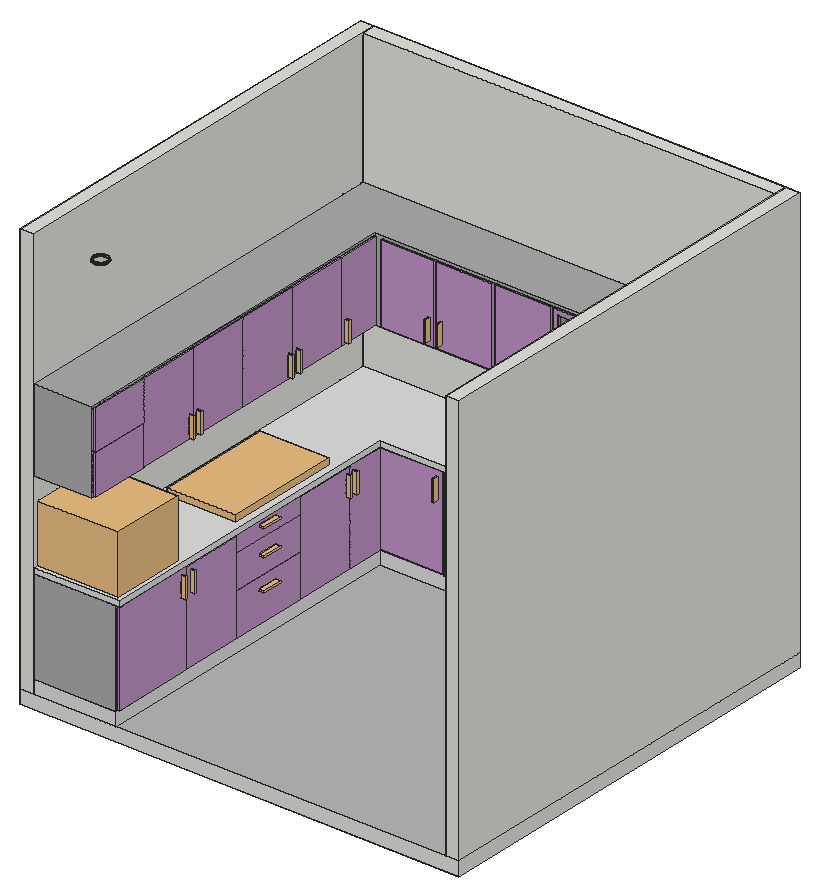
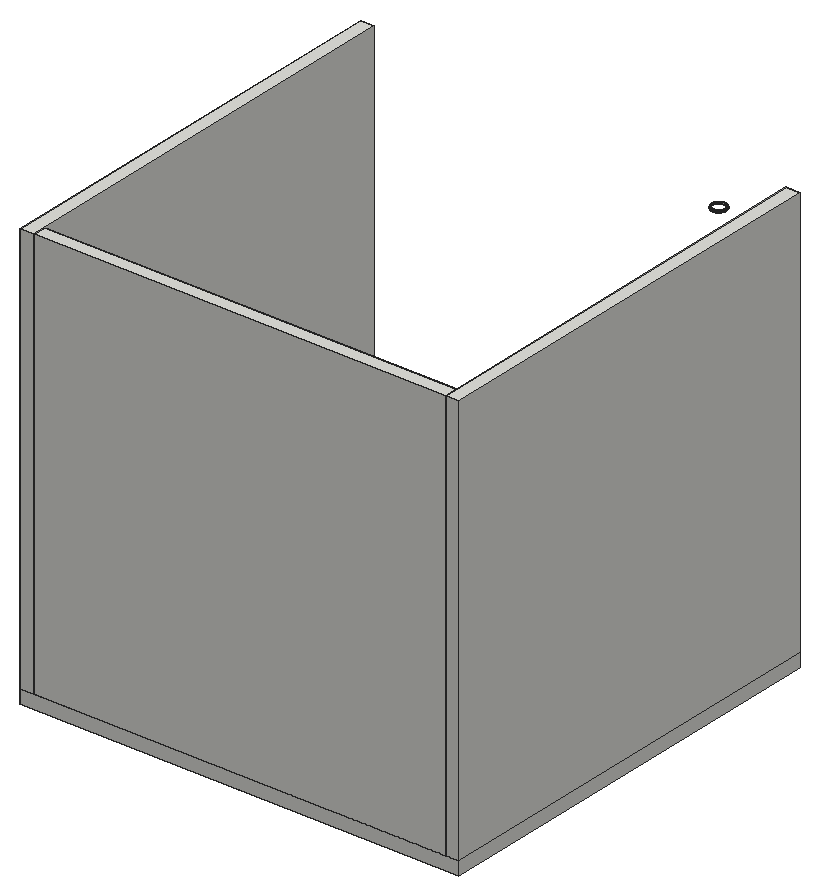
# SketchUp Ruby script. Lengths in inches.
U = 1.inch
M = Sketchup.active_model
def pt(a) = Geom::Point3d.new(a.map { |v| v * U })
def face(e, loops, mat)
  f = e.add_face(loops[0].map { |a| pt(a) })
  loops[1..].each { |l| e.add_face(l.map { |a| pt(a) }).erase! }
  f.material = f.back_material = mat if mat
  f
end
# faces: each face lists its corners as indices into pts; further lists are holes
def faces(e, pts, list, mat = nil) = list.each { |f| face(e, (f[0].is_a?(Array) ? f : [f]).map { |l| l.map { |i| pts[i] } }, mat) }
# xy, xz, yz: faces in a plane at the given z, y or x. An outline is a flat list of corners, or four numbers for a rectangle; further outlines are holes
def ring(l) = l.size == 4 ? [[l[0], l[1]], [l[2], l[1]], [l[2], l[3]], [l[0], l[3]]] : l.each_slice(2).to_a
def flat(e, list, mat, &to3) = list.each { |f| face(e, (f[0].is_a?(Array) ? f : [f]).map { |l| ring(l).map { |u, v| to3.(u, v) } }, mat) }
def xy(e, z, list, mat = nil) = flat(e, list, mat) { |x, y| [x, y, z] }
def xz(e, y, list, mat = nil) = flat(e, list, mat) { |x, z| [x, y, z] }
def yz(e, x, list, mat = nil) = flat(e, list, mat) { |y, z| [x, y, z] }
def lines(e, pts, list) = list.each { |a, b| e.add_line(pt(pts[a]), pt(pts[b])) }
# prism: a flat outline (further loops are holes) pulled along v
def prism(e, loops, v, mat = nil)
  f = face(e, loops, mat); d = Geom::Vector3d.new(v.map { |x| x * U })
  f.pushpull(f.normal.samedirection?(d) ? d.length : -d.length)
end
def box(e, o, s, mat = nil) = prism(e, [[o, [o[0] + s[0], o[1], o[2]], [o[0] + s[0], o[1] + s[1], o[2]], [o[0], o[1] + s[1], o[2]]]], [0, 0, s[2]], mat)
def at(x, y, z, deg = 0) = Geom::Transformation.translation(pt([x, y, z])) * Geom::Transformation.rotation(ORIGIN, Z_AXIS, deg.degrees)
def axes(o, x, y, z) = Geom::Transformation.new([*x, 0, *y, 0, *z, 0, *pt(o).to_a, 1])
def part(name) = M.definitions.add(name)
# library, detail: a bought-in or finely detailed component or shape, given as its bounding box
def library(name, o, s) = part(name).tap { |d| box(d.entities, o, s) }
def detail(e, o, s) = box(e.add_group.entities, o, s)
def put(e, d, t, mat = nil) = e.add_instance(d, t).tap { |i| i.material = mat if mat }
def group(e, t, mat = nil) = e.add_group.tap { |g| g.transformation = t; g.material = mat if mat }.entities
root = M.entities
M.materials.add("Marble White 100cm").color = [222, 222, 222]
M.materials.add("Tiles Simple 02 100cm").color = [183, 183, 183]
M.materials.add("base cabinate colour").color = [192, 148, 199]
M.materials.add("cabinate colour").color = [171, 171, 171]
M.materials.add("clear glass").color = [0, 0, 0]
M.materials["clear glass"].alpha = 0.1
c1 = library("geladeira side by side",[0,0,0],[32.68,30.71,73.23])
c2 = library("9-POIGNEE CLC2",[-3.01,-0.26,0],[6.02,0.52,1.49])
c3 = library("Kitchen sink assembly",[0,0,0],[21.65,23.57,24.55])
c4 = library("Group\#38",[0,0,0],[9.87,6.84,12.32])
c5 = library("7-TABLE DE CUISSON CLC2",[-16.93,-10.04,0.13],[33.86,20.08,1.97])
xy(root,113.9,[[[16.806,6.374,16.577,6.375,16.349,6.4,16.125,6.449,15.907,6.521,15.697,6.616,15.499,6.732,15.315,6.868,15.145,7.023,14.992,7.194,14.858,7.381,14.745,7.58,14.653,7.79,14.583,8.009,14.537,8.234,14.514,8.462,14.515,8.692,14.541,8.92,14.59,9.144,14.662,9.362,14.757,9.571,14.872,9.769,15.008,9.954,15.163,10.124,15.335,10.276,15.521,10.41,15.72,10.524,15.931,10.616,16.149,10.685,16.374,10.732,16.603,10.754,16.832,10.753,17.06,10.728,17.284,10.679,17.502,10.607,17.711,10.512,17.91,10.396,18.094,10.26,18.264,10.105,18.417,9.934,18.551,9.747,18.664,9.548,18.756,9.338,18.826,9.119,18.872,8.894,18.895,8.666,18.894,8.436,18.868,8.208,18.819,7.984,18.747,7.766,18.652,7.557,18.537,7.359,18.4,7.174,18.246,7.004,18.074,6.852,17.888,6.718,17.689,6.604,17.478,6.512,17.26,6.443,17.035,6.396],[16.797,6.573,16.901,6.584,17.005,6.594,17.209,6.636,17.308,6.668,17.408,6.699,17.503,6.741,17.599,6.783,17.689,6.835,17.78,6.886,17.865,6.947,17.949,7.008,18.027,7.077,18.105,7.147,18.176,7.224,18.246,7.301,18.308,7.385,18.369,7.469,18.475,7.649,18.561,7.839,18.594,7.938,18.626,8.037,18.649,8.139,18.671,8.241,18.682,8.344,18.694,8.448,18.695,8.552,18.695,8.657,18.685,8.76,18.675,8.864,18.653,8.966,18.632,9.068,18.601,9.168,18.569,9.267,18.527,9.363,18.485,9.458,18.434,9.549,18.382,9.64,18.321,9.724,18.261,9.809,18.191,9.887,18.122,9.965,17.968,10.105,17.8,10.229,17.71,10.282,17.62,10.334,17.43,10.42,17.232,10.486,17.028,10.53,16.924,10.542,16.82,10.553,16.612,10.555,16.508,10.544,16.404,10.534,16.2,10.492,16.101,10.46,16.001,10.429,15.906,10.387,15.81,10.345,15.72,10.293,15.629,10.242,15.459,10.12,15.382,10.051,15.304,9.981,15.233,9.904,15.163,9.827,15.101,9.743,15.04,9.659,14.934,9.479,14.848,9.289,14.815,9.19,14.783,9.091,14.76,8.989,14.738,8.887,14.727,8.784,14.715,8.68,14.714,8.576,14.714,8.471,14.724,8.368,14.734,8.264,14.755,8.162,14.777,8.06,14.808,7.96,14.84,7.861,14.882,7.765,14.924,7.67,14.975,7.579,15.027,7.488,15.088,7.404,15.148,7.319,15.218,7.241,15.287,7.163,15.441,7.023,15.609,6.899,15.699,6.846,15.789,6.794,15.979,6.708,16.177,6.642,16.381,6.598,16.485,6.586,16.588,6.575,16.693,6.574]],[16.797,6.573,16.693,6.574,16.901,6.584],[16.693,6.574,16.588,6.575,16.485,6.586],[16.901,6.584,17.107,6.615,17.005,6.594],[16.485,6.586,16.381,6.598,16.279,6.62],
  [17.107,6.615,17.308,6.668,17.209,6.636],[16.279,6.62,16.177,6.642,16.078,6.675],[17.308,6.668,17.503,6.741,17.408,6.699],[16.078,6.675,15.979,6.708,15.884,6.751],[17.503,6.741,17.689,6.835,17.599,6.783],
  [15.884,6.751,15.789,6.794,15.699,6.846],[17.689,6.835,17.865,6.947,17.78,6.886],[15.699,6.846,15.609,6.899,15.525,6.961],[17.865,6.947,18.027,7.077,17.949,7.008],[15.525,6.961,15.441,7.023,15.364,7.093],
  [18.027,7.077,18.176,7.224,18.105,7.147],[15.364,7.093,15.287,7.163,15.218,7.241],[18.176,7.224,18.308,7.385,18.246,7.301],[15.218,7.241,15.148,7.319,15.088,7.404],[18.308,7.385,18.422,7.559,18.369,7.469],
  [15.088,7.404,15.027,7.488,14.975,7.579],[18.422,7.559,18.518,7.744,18.475,7.649],[14.975,7.579,14.924,7.67,14.882,7.765],[18.518,7.744,18.594,7.938,18.561,7.839],[14.882,7.765,14.84,7.861,14.808,7.96],
  [18.594,7.938,18.649,8.139,18.626,8.037],[14.808,7.96,14.777,8.06,14.755,8.162],[14.755,8.162,14.734,8.264,14.724,8.368],[14.724,8.368,14.714,8.471,14.714,8.576],[14.714,8.576,14.715,8.68,14.727,8.784],
  [14.727,8.784,14.738,8.887,14.76,8.989],[14.76,8.989,14.783,9.091,14.815,9.19],[14.815,9.19,14.848,9.289,14.891,9.384],[14.891,9.384,14.934,9.479,14.987,9.569],[14.987,9.569,15.04,9.659,15.101,9.743],
  [15.101,9.743,15.163,9.827,15.233,9.904],[15.233,9.904,15.304,9.981,15.382,10.051],[15.382,10.051,15.459,10.12,15.544,10.181],[15.544,10.181,15.629,10.242,15.72,10.293],[15.72,10.293,15.81,10.345,15.906,10.387]])
p = [[16.125,6.449,114],[15.907,6.521,114],[15.907,6.521,113.9],[16.125,6.449,113.9],[16.349,6.4,114],[16.349,6.4,113.9],
  [16.577,6.375,114],[16.577,6.375,113.9],[16.806,6.374,114],[16.806,6.374,113.9],[17.035,6.396,114],[17.035,6.396,113.9],
  [17.26,6.443,114],[17.26,6.443,113.9],[17.478,6.512,114],[17.478,6.512,113.9],[15.697,6.616,114],[15.697,6.616,113.9],
  [17.689,6.604,114],[17.689,6.604,113.9],[15.499,6.732,114],[15.499,6.732,113.9],[16.177,6.642,114.472],[16.177,6.642,113.9],
  [16.078,6.675,113.9],[15.979,6.708,113.9],[15.979,6.708,114.472],[16.381,6.598,114.472],[16.381,6.598,113.9],[16.279,6.62,113.9],
  [16.588,6.575,114.472],[16.588,6.575,113.9],[16.485,6.586,113.9],[16.797,6.573,114.472],[16.797,6.573,113.9],[16.693,6.574,113.9],
  [17.005,6.594,114.472],[17.005,6.594,113.9],[16.901,6.584,113.9],[17.209,6.636,114.472],[17.209,6.636,113.9],[17.107,6.615,113.9],
  [17.408,6.699,114.472],[17.408,6.699,113.9],[17.308,6.668,113.9],[17.888,6.718,114],[17.888,6.718,113.9],[15.315,6.868,114],
  [15.315,6.868,113.9],[15.884,6.751,113.9],[15.789,6.794,113.9],[15.789,6.794,114.472],[17.599,6.783,114.472],[17.599,6.783,113.9],
  [17.503,6.741,113.9],[18.074,6.852,114],[18.074,6.852,113.9],[15.699,6.846,113.9],[15.609,6.899,113.9],[15.609,6.899,114.472],
  [17.78,6.886,114.472],[17.78,6.886,113.9],[17.689,6.835,113.9],[15.145,7.023,114],[15.145,7.023,113.9],[15.525,6.961,113.9],
  [15.441,7.023,113.9],[15.441,7.023,114.472],[17.949,7.008,114.472],[17.949,7.008,113.9],[17.865,6.947,113.9],[18.246,7.004,114],
  [18.246,7.004,113.9],[14.992,7.194,114],[14.992,7.194,113.9],[15.364,7.093,113.9],[15.287,7.163,113.9],[15.287,7.163,114.472],
  [18.105,7.147,114.472],[18.105,7.147,113.9],[18.027,7.077,113.9],[18.4,7.174,114],[18.4,7.174,113.9],[18.246,7.301,114.472],
  [18.246,7.301,113.9],[18.176,7.224,113.9],[14.858,7.381,114],[14.858,7.381,113.9],[15.218,7.241,113.9],[15.148,7.319,113.9],
  [15.148,7.319,114.472],[18.537,7.359,114],[18.537,7.359,113.9],[15.088,7.404,113.9],[15.027,7.488,113.9],[15.027,7.488,114.472],
  [18.369,7.469,114.472],[18.369,7.469,113.9],[18.308,7.385,113.9],[14.745,7.58,114],[14.745,7.58,113.9],[18.652,7.557,114],
  [18.652,7.557,113.9],[14.975,7.579,113.9],[14.924,7.67,113.9],[14.924,7.67,114.472],[18.475,7.649,114.472],[18.475,7.649,113.9],
  [18.422,7.559,113.9],[14.653,7.79,114],[14.653,7.79,113.9],[18.561,7.839,114.472],[18.561,7.839,113.9],[18.518,7.744,113.9],
  [18.747,7.766,114],[18.747,7.766,113.9],[14.882,7.765,113.9],[14.84,7.861,113.9],[14.84,7.861,114.472],[14.583,8.009,114],
  [14.583,8.009,113.9],[18.626,8.037,114.472],[18.626,8.037,113.9],[18.594,7.938,113.9],[18.819,7.984,114],[18.819,7.984,113.9],
  [14.808,7.96,113.9],[14.777,8.06,113.9],[14.777,8.06,114.472],[14.537,8.234,114],[14.537,8.234,113.9],[18.671,8.241,114.472],
  [18.671,8.241,113.9],[18.649,8.139,113.9],[18.868,8.208,114],[18.868,8.208,113.9],[14.755,8.162,113.9],[14.734,8.264,113.9],
  [14.734,8.264,114.472],[14.514,8.462,114],[14.514,8.462,113.9],[18.694,8.448,114.472],[18.694,8.448,113.9],[18.682,8.344,113.9],
  [18.894,8.436,114],[18.894,8.436,113.9],[14.724,8.368,113.9],[14.714,8.471,113.9],[14.714,8.471,114.472],[18.695,8.657,114.472],
  [18.695,8.657,113.9],[18.695,8.552,113.9],[18.895,8.666,114],[18.895,8.666,113.9],[14.515,8.692,114],[14.515,8.692,113.9],
  [14.714,8.576,113.9],[14.715,8.68,113.9],[14.715,8.68,114.472],[14.541,8.92,114],[14.541,8.92,113.9],[14.727,8.784,113.9],
  [14.738,8.887,113.9],[14.738,8.887,114.472],[18.675,8.864,114.472],[18.675,8.864,113.9],[18.685,8.76,113.9],[18.872,8.894,114],
  [18.872,8.894,113.9],[14.59,9.144,114],[14.59,9.144,113.9],[14.76,8.989,113.9],[14.783,9.091,113.9],[14.783,9.091,114.472],
  [18.632,9.068,114.472],[18.632,9.068,113.9],[18.653,8.966,113.9],[18.826,9.119,114],[18.826,9.119,113.9],[14.662,9.362,114],
  [14.662,9.362,113.9],[14.815,9.19,113.9],[14.848,9.289,113.9],[14.848,9.289,114.472],[18.569,9.267,114.472],[18.569,9.267,113.9],
  [18.601,9.168,113.9],[18.756,9.338,114],[18.756,9.338,113.9],[14.891,9.384,113.9],[14.934,9.479,113.9],[14.934,9.479,114.472],
  [18.485,9.458,114.472],[18.485,9.458,113.9],[18.527,9.363,113.9],[18.664,9.548,114],[18.664,9.548,113.9],[14.757,9.571,114],
  [14.757,9.571,113.9],[14.987,9.569,113.9],[15.04,9.659,113.9],[15.04,9.659,114.472],[18.382,9.64,114.472],[18.382,9.64,113.9],
  [18.434,9.549,113.9],[18.551,9.747,114],[18.551,9.747,113.9],[14.872,9.769,114],[14.872,9.769,113.9],[18.261,9.809,114.472],
  [18.261,9.809,113.9],[18.321,9.724,113.9],[15.101,9.743,113.9],[15.163,9.827,113.9],[15.163,9.827,114.472],[18.417,9.934,114],
  [18.417,9.934,113.9],[15.008,9.954,114],[15.008,9.954,113.9],[15.233,9.904,113.9],[15.304,9.981,113.9],[15.304,9.981,114.472],
  [18.122,9.965,114.472],[18.122,9.965,113.9],[18.191,9.887,113.9],[18.264,10.105,114],[18.264,10.105,113.9],[15.163,10.124,114],
  [15.163,10.124,113.9],[15.382,10.051,113.9],[15.459,10.12,113.9],[15.459,10.12,114.472],[17.968,10.105,114.472],[17.968,10.105,113.9],
  [18.045,10.035,113.9],[15.335,10.276,114],[15.335,10.276,113.9],[15.544,10.181,113.9],[15.629,10.242,113.9],[15.629,10.242,114.472],
  [17.8,10.229,114.472],[17.8,10.229,113.9],[17.884,10.167,113.9],[18.094,10.26,114],[18.094,10.26,113.9],[15.72,10.293,113.9],
  [15.81,10.345,113.9],[15.81,10.345,114.472],[17.62,10.334,114.472],[17.62,10.334,113.9],[17.71,10.282,113.9],[15.521,10.41,114],
  [15.521,10.41,113.9],[15.906,10.387,113.9],[16.001,10.429,113.9],[16.001,10.429,114.472],[17.43,10.42,114.472],[17.43,10.42,113.9],
  [17.525,10.377,113.9],[17.91,10.396,114],[17.91,10.396,113.9],[15.72,10.524,114],[15.72,10.524,113.9],[16.101,10.46,113.9],
  [16.2,10.492,113.9],[16.2,10.492,114.472],[17.232,10.486,114.472],[17.232,10.486,113.9],[17.331,10.453,113.9],[17.711,10.512,114],
  [17.711,10.512,113.9],[15.931,10.616,114],[15.931,10.616,113.9],[16.302,10.513,113.9],[16.404,10.534,113.9],[16.404,10.534,114.472],
  [16.508,10.544,113.9],[16.612,10.555,113.9],[16.612,10.555,114.472],[16.82,10.553,114.472],[16.82,10.553,113.9],[16.924,10.542,113.9],
  [17.028,10.53,113.9],[17.028,10.53,114.472],[17.13,10.508,113.9],[17.502,10.607,114],[17.502,10.607,113.9],[16.149,10.685,114],
  [16.149,10.685,113.9],[16.716,10.554,113.9],[17.284,10.679,114],[17.284,10.679,113.9],[16.374,10.732,114],[16.374,10.732,113.9],
  [16.603,10.754,114],[16.603,10.754,113.9],[16.832,10.753,114],[17.06,10.728,114],[17.06,10.728,113.9],[16.832,10.753,113.9],
  [4,120,0],[4,0,0],[124,0,0],[124,120,0],[21,0.709,80.362],[21,0,80.362],
  [94.291,103,80.362],[95,103,80.362]]
faces(root,p,[[0,1,2,3],[4,0,3,5],[6,4,5,7],[8,6,7,9],[10,8,9,11],[12,10,11,13],[14,12,13,15],[1,16,17,2],
  [18,14,15,19],[16,20,21,17],[22,23,24,25,26],[27,28,29,23,22],[30,31,32,28,27],[33,34,35,31,30],[36,37,38,34,33],[39,40,41,37,36],
  [42,43,44,40,39],[45,18,19,46],[20,47,48,21],[26,25,49,50,51],[52,53,54,43,42],[55,45,46,56],[51,50,57,58,59],[60,61,62,53,52],
  [47,63,64,48],[59,58,65,66,67],[68,69,70,61,60],[71,55,56,72],[63,73,74,64],[67,66,75,76,77],[78,79,80,69,68],[81,71,72,82],
  [83,84,85,79,78],[73,86,87,74],[77,76,88,89,90],[91,81,82,92],[90,89,93,94,95],[96,97,98,84,83],[86,99,100,87],[101,91,92,102],
  [95,94,103,104,105],[106,107,108,97,96],[99,109,110,100],[111,112,113,107,106],[114,101,102,115],[105,104,116,117,118],[109,119,120,110],[121,122,123,112,111],
  [124,114,115,125],[118,117,126,127,128],[119,129,130,120],[131,132,133,122,121],[134,124,125,135],[128,127,136,137,138],[129,139,140,130],[141,142,143,132,131],
  [144,134,135,145],[138,137,146,147,148],[149,150,151,142,141],[152,144,145,153],[139,154,155,140],[148,147,156,157,158],[154,159,160,155],[158,157,161,162,163],
  [164,165,166,150,149],[167,152,153,168],[159,169,170,160],[163,162,171,172,173],[174,175,176,165,164],[177,167,168,178],[169,179,180,170],[173,172,181,182,183],
  [184,185,186,175,174],[187,177,178,188],[183,182,189,190,191],[192,193,194,185,184],[195,187,188,196],[179,197,198,180],[191,190,199,200,201],[202,203,204,193,192],
  [205,195,196,206],[197,207,208,198],[209,210,211,203,202],[201,200,212,213,214],[215,205,206,216],[207,217,218,208],[214,213,219,220,221],[222,223,224,210,209],
  [225,215,216,226],[217,227,228,218],[221,220,229,230,231],[232,233,234,223,222],[227,235,236,228],[231,230,237,238,239],[240,241,242,233,232],[243,225,226,244],
  [239,238,245,246,247],[248,249,250,241,240],[235,251,252,236],[247,246,253,254,255],[256,257,258,249,248],[259,243,244,260],[251,261,262,252],[255,254,263,264,265],
  [266,267,268,257,256],[269,259,260,270],[261,271,272,262],[265,264,273,274,275],[275,274,276,277,278],[279,280,281,282,283],[283,282,284,267,266],[285,269,270,286],
  [271,287,288,272],[278,277,289,280,279],[290,285,286,291],[287,292,293,288],[292,294,295,293],[296,297,298,299],[297,290,291,298],[294,296,299,295]])
lines(root,p,[[300,301],[302,303],[303,300],[304,305],[306,307]])
g1 = group(root,at(0,0,-4))
xy(g1,0,[[0,0,128,124]])
xy(g1,4,[[0,0,128,124]],"Tiles Simple 02 100cm")
xz(g1,0,[[0,0,128,4]])
xz(g1,124,[[0,0,128,4]])
yz(g1,0,[[0,0,124,4]])
yz(g1,128,[[0,0,124,4]])
put(root,c1,axes([96.28,95.43,0],[0.8,0,0],[0,0.8,0],[0,0,0.8]))
g2 = group(root,at(124,-4,0))
box(g2,[0,4,0],[4,124,120])
g3 = group(root,at(4,120,0))
box(g3,[0,0,0],[120,4,120])
g4 = group(root,at(0,-4,0))
box(g4,[0,4,0],[4,124,120])
g5 = group(root,at(4,0,0),"Marble White 100cm")
prism(g5,[[[24,96,0],[24,0,0],[0,0,0],[0,120,0],[91,120,0],[91,96,0]]],[0,0,3.9375])
g6 = group(root,at(4,0,3.9375),"cabinate colour")
xy(g6,0,[[0,0,0,120,91,120,91,96,24,96,24,0]])
xy(g6,0.71,[[0,0.71,24,24.33],[0,25.04,24,42.33],[0,43.04,24,65.95],[0,66.66,24,83.95],[0,84.66,24,84.66,24,95.09,22.47,95.09,22.47,120,0,120],
  [24.71,96,42.71,118.83],[43.42,96,60.71,119.03],[61.42,96,78.71,119.03],[79.42,96,90.29,119.03]])
xy(g6,12.36,[[0,43.04,24,65.95]])
xy(g6,13.07,[[0,43.04,24,65.95]])
xy(g6,22.2,[[0,43.04,24,65.95]])
xy(g6,22.91,[[0,43.04,24,65.95]])
xy(g6,26.85,[[0,25.04,24,42.33],[0,43.04,24,65.95],[0,66.66,24,83.95],[0,84.66,0,120,22.47,120,22.47,95.09,24,95.09,24,84.66],[24.71,96,42.71,118.83],
  [43.42,96,60.71,119.03],[61.42,96,78.71,119.03],[79.42,96,90.29,119.03]])
xy(g6,27.56,[[[0,0,24,0,24,96,91,96,91,120,0,120],[8.17,2.03,8.01,2.1,7.96,2.125,7.84,2.24,7.8,2.28,7.73,2.4375,7.71,2.49,7.71,21.81,7.78,21.97,7.8,22.02,7.91,22.14,7.96,22.18,8.11,22.25,8.17,22.27,22.4375,22.27,22.6,22.2,22.65,22.18,22.77,22.0625,22.81,22.02,22.875,21.87,22.9,21.81,22.9,2.49,22.83,2.34,22.81,2.28,22.69,2.16,22.65,2.125,22.49,2.06,22.4375,2.03]]])
xz(g6,0,[[0,0,24,27.56]])
xz(g6,0.71,[[0,0.71,24,26.85]])
xz(g6,24.33,[[0,0.71,24,26.85]])
xz(g6,25.04,[[0,0.71,24,26.85]])
xz(g6,42.33,[[0,0.71,24,26.85]])
xz(g6,43.04,[[0,0.71,24,12.36],[0,13.07,24,22.2],[0,22.91,24,26.85]])
xz(g6,65.95,[[0,0.71,24,12.36],[0,13.07,24,22.2],[0,22.91,24,26.85]])
xz(g6,66.66,[[0,0.71,24,26.85]])
xz(g6,83.95,[[0,0.71,24,26.85]])
xz(g6,84.66,[[0,0.71,24,26.85]])
xz(g6,95.09,[[22.47,0.71,24,26.85]])
xz(g6,96,[[24,0,91,0,91,26.85,90.29,26.85,90.29,0.71,24.71,0.71,24.71,26.85,24,26.85],[42.71,0.71,43.42,26.85],[60.71,0.71,61.42,26.85],[78.71,0.71,79.42,26.85],[24,26.85,91,27.56]])
xz(g6,118.83,[[24.71,0.71,42.71,26.85]])
xz(g6,119.03,[[43.42,0.71,60.71,26.85],[61.42,0.71,78.71,26.85],[79.42,0.71,90.29,26.85]])
xz(g6,120,[[0,0,0,0.71,22.47,0.71,22.47,26.85,0,26.85,0,27.56,91,27.56,91,0]])
yz(g6,0,[[[0,0,0,27.56,120,27.56,120,26.85,84.66,26.85,84.66,0.71,120,0.71,120,0],[0.71,0.71,24.33,26.85],[66.66,0.71,83.95,26.85],[25.04,0.71,42.33,26.85],[43.04,0.71,65.95,12.36],[43.04,13.07,65.95,22.2],[43.04,22.91,65.95,26.85]]])
yz(g6,22.47,[[95.09,0.71,120,26.85]])
yz(g6,24,[[0,0,96,0,96,26.85,95.09,26.85,95.09,0.71,0.71,0.71,0.71,26.85,0,26.85],[24.33,0.71,25.04,26.85],[42.33,0.71,43.04,26.85],[65.95,0.71,66.66,26.85],[83.95,0.71,84.66,26.85],
  [43.04,12.36,65.95,13.07],[43.04,22.2,65.95,22.91],[0,26.85,96,27.56]])
yz(g6,24.71,[[96,0.71,118.83,26.85]])
yz(g6,42.71,[[96,0.71,118.83,26.85]])
yz(g6,43.42,[[96,0.71,119.03,26.85]])
yz(g6,60.71,[[96,0.71,119.03,26.85]])
yz(g6,61.42,[[96,0.71,119.03,26.85]])
yz(g6,78.71,[[96,0.71,119.03,26.85]])
yz(g6,79.42,[[96,0.71,119.03,26.85]])
yz(g6,90.29,[[96,0.71,119.03,26.85]])
yz(g6,91,[[96,0,120,27.56]])
g7 = group(root,at(28,0.35,4.29),"base cabinate colour")
box(g7,[0,0,0],[0.71,24.23,26.85])
box(g7,[0,24.43,0],[0.71,17.8,26.85])
box(g7,[0,42.43,22.2],[0.71,23.42,4.65])
box(g7,[0,42.43,12.46],[0.71,23.42,9.65])
box(g7,[0,42.43,0],[0.71,23.42,12.26])
box(g7,[0,66.05,0],[0.71,17.8,26.85])
box(g7,[0,84.05,0],[0.71,11.14,26.85])
g8 = group(root,at(47.16,95.29,4.29),"base cabinate colour")
box(g8,[0,0,0],[17.8,0.71,26.85])
g9 = group(root,at(65.16,95.29,4.29),"base cabinate colour")
box(g9,[0,0,0],[17.8,0.71,26.85])
g10 = group(root,at(83.16,95.29,4.29),"base cabinate colour")
box(g10,[0,0,0],[11.39,0.71,26.85])
g11 = group(root,at(28.71,95.29,4.65),"base cabinate colour")
box(g11,[0,0,0],[18.26,0.71,26.5])
put(root,c2,axes([28.71,54.19,13.52],[0,1,0],[0,0,1],[1,0,0]))
put(root,c2,axes([28.71,54.19,22.49],[0,1,0],[0,0,1],[1,0,0]))
put(root,c2,axes([45.3,95.29,26.47],[0,0,-1],[1,0,0],[0,-1,0]))
put(root,c2,axes([49.22,95.29,26.47],[0,0,-1],[1,0,0],[0,-1,0]))
put(root,c2,axes([81.68,95.29,26.47],[0,0,-1],[1,0,0],[0,-1,0]))
put(root,c2,axes([84.24,95.29,26.47],[0,0,-1],[1,0,0],[0,-1,0]))
put(root,c2,axes([28.71,22.89,26.9],[0,0,-1],[0,1,0],[1,0,0]))
put(root,c2,axes([28.71,26.22,26.9],[0,0,-1],[0,1,0],[1,0,0]))
put(root,c2,axes([28.71,82.96,26.9],[0,0,-1],[0,1,0],[1,0,0]))
put(root,c2,axes([28.71,85.27,26.9],[0,0,-1],[0,1,0],[1,0,0]))
put(root,c3,at(27.57,1.32,25.41,90))
put(root,c2,axes([28.71,54.19,30.17],[0,1,0],[0,0,1],[1,0,0]))
g12 = group(root,at(4,0,31.5),"Marble White 100cm")
xy(g12,0,[[[0,0,0,120,91,120,91,96,24,96,24,0],[8.169,2.035,22.438,2.035,22.494,2.058,22.651,2.123,22.808,2.28,22.832,2.336,22.897,2.493,22.897,21.81,22.874,21.866,22.808,22.023,22.651,22.18,22.595,22.203,22.438,22.269,8.169,22.269,8.113,22.245,7.956,22.18,7.799,22.023,7.776,21.967,7.71,21.81,7.71,2.493,7.734,2.4375,7.799,2.28,7.956,2.123,8.011,2.1]],[24,0,24,96,91,96,91,95.016,24.984,95.016,24.984,0]],"Marble White 100cm")
xy(g12,1.575,[[[0,0,24.984,0,24.984,95.016,91,95.016,91,120,0,120],[8.169,2.035,7.96,2.121,7.956,2.123,7.799,2.28,7.712,2.489,7.71,2.493,7.71,21.81,7.797,22.018,7.799,22.023,7.952,22.177,7.956,22.18,8.164,22.267,8.169,22.269,22.438,22.269,22.646,22.182,22.651,22.18,22.808,22.023,22.895,21.814,22.897,21.81,22.897,2.493,22.81,2.285,22.808,2.28,22.651,2.123,22.442,2.036,22.438,2.035]]],"Marble White 100cm")
xz(g12,0,[[0,0,24.984,1.575]],"Marble White 100cm")
xz(g12,95.016,[[24.984,0,91,1.575]],"Marble White 100cm")
xz(g12,120,[[0,0,91,1.575]],"Marble White 100cm")
yz(g12,0,[[0,0,120,1.575]],"Marble White 100cm")
yz(g12,24.984,[[0,0,95.016,1.575]],"Marble White 100cm")
yz(g12,91,[[95.016,0,120,1.575]],"Marble White 100cm")
put(root,c4,axes([84.41,119.08,33.07],[0,-1.33,0],[1.33,0,0],[0,0,1.33]))
put(root,c5,at(16.99,61.9,33.07,90))
g13 = group(root,at(4,0,57.07),"cabinate colour")
xy(g13,0,[[0,0,0,120,91,120,91,103,17,103,17,0]])
xy(g13,0.71,[[0,0.71,17,17.71],[0,18.42,17,35.71],[0,36.42,17,53.71],[0,54.42,17,71.71],[0,72.42,17,89.71],
  [0,90.42,17,90.42,17,102.29,15.86,102.29,15.86,120,0,120],[19.26,103,34.71,120],[35.42,103,51.71,120],[52.42,103,68.71,120],[69.42,103,90.29,120]])
xy(g13,11.65,[[0,0.71,16.02,17.71],[69.42,103.98,90.29,120]])
xy(g13,12.35,[[0,0.71,16.02,17.71],[69.42,103.98,90.29,120]])
xy(g13,23.29,[[0,0.71,17,17.71],[0,18.42,17,35.71],[0,36.42,17,53.71],[0,54.42,17,71.71],[0,72.42,17,89.71],
  [0,90.42,0,120,15.86,120,15.86,102.29,17,102.29,17,90.42],[19.26,103,34.71,120],[35.42,103,51.71,120],[52.42,103,68.71,120],[69.42,103,90.29,120]])
xy(g13,24,[[0,0,17,0,17,103,91,103,91,120,0,120]])
xz(g13,0,[[0,0,17,24]])
xz(g13,0.71,[[0,0.71,17,11.65],[16.02,11.65,17,12.35],[0,12.35,17,23.29]])
xz(g13,17.71,[[0,0.71,17,11.65],[16.02,11.65,17,12.35],[0,12.35,17,23.29]])
xz(g13,18.42,[[0,0.71,17,23.29]])
xz(g13,35.71,[[0,0.71,17,23.29]])
xz(g13,36.42,[[0,0.71,17,23.29]])
xz(g13,53.71,[[0,0.71,17,23.29]])
xz(g13,54.42,[[0,0.71,17,23.29]])
xz(g13,71.71,[[0,0.71,17,23.29]])
xz(g13,72.42,[[0,0.71,17,23.29]])
xz(g13,89.71,[[0,0.71,17,23.29]])
xz(g13,90.42,[[0,0.71,17,23.29]])
xz(g13,102.29,[[15.86,0.71,17,23.29]])
xz(g13,103,[[[17,0,91,24],[19.26,0.71,90.29,23.29]],[34.71,0.71,35.42,23.29],[51.71,0.71,52.42,23.29],[68.71,0.71,69.42,23.29]])
xz(g13,103.98,[[69.42,11.65,90.29,12.35]])
xz(g13,120,[[[0,0,0,0.71,15.86,0.71,15.86,23.29,0,23.29,0,24,91,24,91,0],[52.42,0.71,68.71,23.29],[35.42,0.71,51.71,23.29],[19.26,0.71,34.71,23.29],[69.42,0.71,90.29,11.65],[69.42,12.35,90.29,23.29]]])
yz(g13,0,[[[0,0,0,24,120,24,120,23.29,90.42,23.29,90.42,0.71,120,0.71,120,0],[36.42,0.71,53.71,23.29],[54.42,0.71,71.71,23.29],[72.42,0.71,89.71,23.29],[18.42,0.71,35.71,23.29],[0.71,12.35,17.71,23.29],[0.71,0.71,17.71,11.65]]])
yz(g13,15.86,[[102.29,0.71,120,23.29]])
yz(g13,16.02,[[0.71,11.65,17.71,12.35]])
yz(g13,17,[[[0,0,103,24],[72.42,0.71,89.71,23.29],[54.42,0.71,71.71,23.29],[36.42,0.71,53.71,23.29],[18.42,0.71,35.71,23.29],[0.71,0.71,17.71,23.29],[90.42,0.71,102.29,23.29]]])
yz(g13,19.26,[[103,0.71,120,23.29]])
yz(g13,34.71,[[103,0.71,120,23.29]])
yz(g13,35.42,[[103,0.71,120,23.29]])
yz(g13,51.71,[[103,0.71,120,23.29]])
yz(g13,52.42,[[103,0.71,120,23.29]])
yz(g13,68.71,[[103,0.71,120,23.29]])
yz(g13,69.42,[[103,0.71,120,11.65],[103,11.65,103.98,12.35],[103,12.35,120,23.29]])
yz(g13,90.29,[[103,0.71,120,11.65],[103,11.65,103.98,12.35],[103,12.35,120,23.29]])
yz(g13,91,[[103,0,120,24]])
g14 = group(root,at(21,0.45,69.17),"base cabinate colour")
box(g14,[0,0,0],[0.71,17.51,11.45])
box(g14,[0,0,-11.65],[0.71,17.51,11.45])
box(g14,[0,17.71,-11.65],[0.71,17.8,23.1])
box(g14,[0,35.71,-11.65],[0.71,17.84,23.1])
box(g14,[0,53.75,-11.65],[0.71,17.75,23.1])
box(g14,[0,71.7,-11.65],[0.71,17.81,23.1])
box(g14,[0,89.71,-11.65],[0.71,12.48,23.1])
box(g14,[2.26,101.84,-11.39],[15.45,0.71,22.58])
box(g14,[18.42,101.84,-11.39],[16.29,0.71,22.58])
box(g14,[35.42,101.84,-11.39],[16.29,0.71,22.58])
xy(g14,-11.39,[[52.42,101.84,73.29,102.55]])
xy(g14,-9.89,[[53.92,101.84,71.79,102.19],[53.92,102.19,71.79,102.55]])
xy(g14,9.69,[[53.92,101.84,71.79,102.19],[53.92,102.19,71.79,102.55]])
xy(g14,11.19,[[52.42,101.84,73.29,102.55]])
xz(g14,101.84,[[[52.42,-11.39,73.29,11.19],[53.92,-9.89,71.79,9.69]]])
xz(g14,102.55,[[[52.42,-11.39,73.29,11.19],[53.92,-9.89,71.79,9.69]]])
yz(g14,52.42,[[101.84,-11.39,102.55,11.19]])
yz(g14,53.92,[[101.84,-9.89,102.19,9.69],[102.19,-9.89,102.55,9.69]])
yz(g14,71.79,[[101.84,-9.89,102.19,9.69],[102.19,-9.89,102.55,9.69]])
yz(g14,73.29,[[101.84,-11.39,102.55,11.19]])
g15 = group(g14,at(53.92,102.19,-9.89),"clear glass")
xz(g15,0,[[0,0,17.875,19.58]])
put(root,c2,axes([21.71,34.62,61.15],[0,0,-1],[0,1,0],[1,0,0]))
put(root,c2,axes([21.71,37.28,61.15],[0,0,-1],[0,1,0],[1,0,0]))
put(root,c2,axes([21.71,70.62,61.15],[0,0,-1],[0,1,0],[1,0,0]))
put(root,c2,axes([21.71,73.54,61.15],[0,0,-1],[0,1,0],[1,0,0]))
put(root,c2,axes([21.71,91.22,61.15],[0,0,-1],[0,1,0],[1,0,0]))
put(root,c2,axes([71.69,102.29,62.15],[0,0,-1],[1,0,0],[0,-1,0]))
put(root,c2,axes([40.77,102.29,62.15],[0,0,-1],[1,0,0],[0,-1,0]))
put(root,c2,axes([37.31,102.29,62.15],[0,0,-1],[1,0,0],[0,-1,0]))
